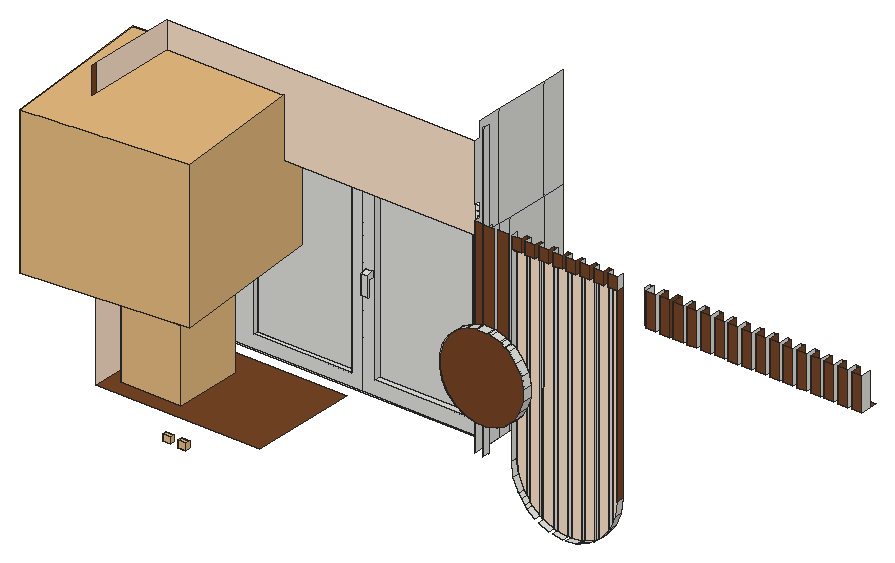
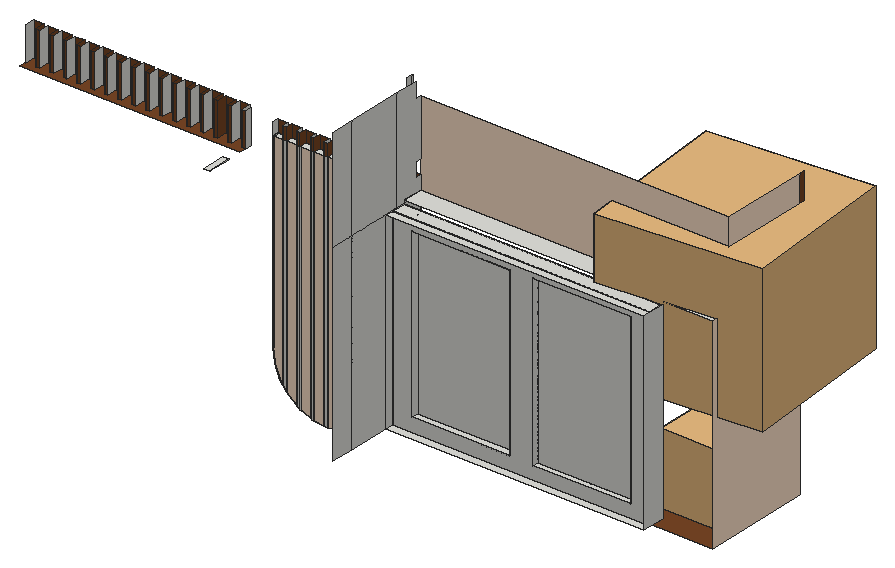
# SketchUp Ruby script. Lengths in inches.
U = 1.inch
M = Sketchup.active_model
def pt(a) = Geom::Point3d.new(a.map { |v| v * U })
def face(e, loops, mat)
  f = e.add_face(loops[0].map { |a| pt(a) })
  loops[1..].each { |l| e.add_face(l.map { |a| pt(a) }).erase! }
  f.material = f.back_material = mat if mat
  f
end
# faces: each face lists its corners as indices into pts; further lists are holes
def faces(e, pts, list, mat = nil) = list.each { |f| face(e, (f[0].is_a?(Array) ? f : [f]).map { |l| l.map { |i| pts[i] } }, mat) }
# xy, xz, yz: faces in a plane at the given z, y or x. An outline is a flat list of corners, or four numbers for a rectangle; further outlines are holes
def ring(l) = l.size == 4 ? [[l[0], l[1]], [l[2], l[1]], [l[2], l[3]], [l[0], l[3]]] : l.each_slice(2).to_a
def flat(e, list, mat, &to3) = list.each { |f| face(e, (f[0].is_a?(Array) ? f : [f]).map { |l| ring(l).map { |u, v| to3.(u, v) } }, mat) }
def xy(e, z, list, mat = nil) = flat(e, list, mat) { |x, y| [x, y, z] }
def xz(e, y, list, mat = nil) = flat(e, list, mat) { |x, z| [x, y, z] }
def yz(e, x, list, mat = nil) = flat(e, list, mat) { |y, z| [x, y, z] }
def lines(e, pts, list) = list.each { |a, b| e.add_line(pt(pts[a]), pt(pts[b])) }
# prism: a flat outline (further loops are holes) pulled along v
def prism(e, loops, v, mat = nil)
  f = face(e, loops, mat); d = Geom::Vector3d.new(v.map { |x| x * U })
  f.pushpull(f.normal.samedirection?(d) ? d.length : -d.length)
end
def box(e, o, s, mat = nil) = prism(e, [[o, [o[0] + s[0], o[1], o[2]], [o[0] + s[0], o[1] + s[1], o[2]], [o[0], o[1] + s[1], o[2]]]], [0, 0, s[2]], mat)
def at(x, y, z, deg = 0) = Geom::Transformation.translation(pt([x, y, z])) * Geom::Transformation.rotation(ORIGIN, Z_AXIS, deg.degrees)
def axes(o, x, y, z) = Geom::Transformation.new([*x, 0, *y, 0, *z, 0, *pt(o).to_a, 1])
def part(name) = M.definitions.add(name)
# library, detail: a bought-in or finely detailed component or shape, given as its bounding box
def library(name, o, s) = part(name).tap { |d| box(d.entities, o, s) }
def detail(e, o, s) = box(e.add_group.entities, o, s)
def put(e, d, t, mat = nil) = e.add_instance(d, t).tap { |i| i.material = mat if mat }
def group(e, t, mat = nil) = e.add_group.tap { |g| g.transformation = t; g.material = mat if mat }.entities
root = M.entities
M.materials.add("[Color C01]").color = [255, 229, 204]
M.materials.add("[Color M02]").color = [198, 198, 198]
M.materials.add("[Color M08]1").color = [30, 30, 30]
M.materials.add("[Wood Veneer 01]").color = [120, 70, 37]
c1 = library("Recessed spotlight",[0,0,0],[1.29,1.0625,0.73])
c2 = part("Window (3)")
xy(c2.entities,31.72,[[-0.78,88.6,2.72,128.1]])
xy(c2.entities,34.95,[[-0.78,91.53,0.84,106.59],[0.84,91.53,1.05,97.58],[1.05,91.53,1.42,106.59],[1.42,91.53,2.72,106.59],[0.84,97.58,1.05,98.18],
  [0.84,98.18,1.05,106.59]])
xy(c2.entities,35.27,[[-0.78,110.09,0.97,125.14],[1.05,110.09,2.72,125.14]])
xy(c2.entities,58.35,[[2.72,108.74,3.8,109.74]])
xy(c2.entities,77.8125,[[-0.78,110.09,2.72,125.14],[0.97,110.09,1.05,125.14]])
xy(c2.entities,77.93,[[-0.78,91.53,0.84,106.59],[1.05,91.53,1.42,106.59],[1.42,91.53,2.72,106.59]])
xy(c2.entities,80.72,[[-0.78,88.6,2.72,128.1]])
xz(c2.entities,88.6,[[-0.78,31.72,2.72,80.72]])
xz(c2.entities,91.53,[[-0.78,34.95,0.84,77.93],[1.05,34.95,1.42,77.93],[1.42,34.95,2.72,77.93]])
xz(c2.entities,106.59,[[-0.78,34.95,0.84,77.93],[0.84,34.95,1.05,77.93],[0.84,34.95,2.72,77.93]])
xz(c2.entities,108.74,[[3.8,54.35,4.22,54.6,4.22,59.47,2.72,59.97,2.72,58.35,3.8,58.35]])
xz(c2.entities,109.74,[[3.8,54.35,3.8,58.35,2.72,58.35,2.72,59.97,4.22,59.47,4.22,54.6]])
xz(c2.entities,110.09,[[-0.78,35.27,0.97,77.8125],[1.05,35.27,2.72,77.8125]])
xz(c2.entities,125.14,[[-0.78,35.27,0.97,77.8125],[0.97,35.27,1.05,80.72],[1.05,35.27,2.72,77.8125]])
xz(c2.entities,128.1,[[-0.78,31.72,2.72,80.72]])
yz(c2.entities,-0.78,[[[88.6,31.72,128.1,80.72],[91.53,34.95,106.59,77.93],[110.09,35.27,125.14,77.8125]]])
yz(c2.entities,0.84,[[91.53,34.95,106.59,77.93]])
yz(c2.entities,0.97,[[110.09,35.27,125.14,77.8125]])
yz(c2.entities,1.05,[[91.53,34.95,106.59,77.93],[110.09,35.27,125.14,77.8125]])
yz(c2.entities,1.42,[[91.53,34.95,106.59,77.93]])
yz(c2.entities,2.72,[[[88.6,31.72,108.35,80.72],[91.53,34.95,106.59,77.93]],[[108.35,31.72,128.1,80.72],[110.09,35.27,125.14,77.8125],[108.74,58.35,109.74,59.97]]])
yz(c2.entities,3.8,[[108.74,54.35,109.74,58.35]])
yz(c2.entities,4.22,[[108.74,54.6,109.74,59.47]])
p = [[4.22,108.74,54.6],[3.8,108.74,54.35],[3.8,109.74,54.35],[4.22,109.74,54.6],[2.72,109.74,59.97],[2.72,108.74,59.97],
  [4.22,108.74,59.47],[4.22,109.74,59.47],[-0.78,86.4,89.94],[-0.78,86.44,89.94],[15.22,130.69,89.94],[15.22,130.65,89.94],
  [-0.78,86.44,28.19],[-0.78,86.4,28.19],[7.72,130.69,89.94],[7.72,130.65,89.94]]
faces(c2.entities,p,[[0,1,2,3],[4,5,6,7]])
lines(c2.entities,p,[[8,9],[10,11],[12,13],[14,15]])
c3 = library("Potted plant pair",[-0.125,-0.11,0],[4.84,5.4,5.74])
c4 = library("Potted trailing plant",[-13.52,-13.75,-7.41],[40.56,40.5625,37.31])
xy(root,46.25,[[6.1,124.71,47.85,152.4]],"[Wood Veneer 01]")
xy(root,48.58,[[18.99,152.4,84.82,158.375]])
xy(root,50.17,[[94.24,147.02,94.43,148.71],[121.11,147.02,121.3,148.65],[121.11,148.65,121.3,148.71]])
xy(root,57.34,[[87.07,144.77,87.24,147.02]])
xy(root,91.72,[[129.68,152.25,131.15,158.375]])
xy(root,93.09,[[129.24,146.15,129.24,148.71,128.3,148.71,128.3,150.65,184.3,150.65,184.3,146.15,181.74,146.15,181.74,148.71,180.8,148.71,180.8,146.15,178.24,146.15,178.24,148.71,177.3,148.71,177.3,146.15,174.74,146.15,174.74,148.71,173.8,148.71,173.8,146.15,171.24,146.15,171.24,148.71,170.3,148.71,170.3,146.15,167.74,146.15,167.74,148.71,166.8,148.71,166.8,146.15,164.24,146.15,164.24,148.71,163.3,148.71,163.3,146.15,160.74,146.15,160.74,148.71,159.8,148.71,159.8,146.15,157.24,146.15,157.24,148.71,156.3,148.71,156.3,146.15,153.74,146.15,153.74,148.71,152.8,148.71,152.8,146.15,150.24,146.15,150.24,148.71,149.3,148.71,149.3,146.15,146.74,146.15,146.74,148.71,145.8,148.71,145.8,146.15,143.24,146.15,143.24,148.71,142.3,148.71,142.3,146.15,139.74,146.15,139.74,148.71,138.8,148.71,138.8,146.15,136.24,146.15,136.24,148.71,135.3,148.71,135.3,146.15,132.74,146.15,132.74,148.71,131.8,148.71,131.8,146.15]],"[Wood Veneer 01]")
xy(root,97.46,[[18.99,152.4,84.82,158.375]])
xy(root,98.3,[[6.1,147.26,84.82,152.4]])
xy(root,98.3,[[6.1,123.26,18.91,147.26]],"[Wood Veneer 01]")
xy(root,98.47,[[94.24,147.02,94.43,148.71],[94.43,147.02,96.8,148.65],[97.74,147.02,100.3,148.65],[101.24,147.02,103.8,148.65],[104.74,147.02,107.3,148.65],
  [108.24,147.02,110.8,148.65],[111.74,147.02,114.3,148.65],[115.24,147.02,117.8,148.65],[118.74,147.02,121.11,148.65],[121.11,147.02,121.3,148.71]])
xy(root,100.37,[[6.1,123.26,18.91,124.71],[6.1,124.71,18.91,147.26]])
xz(root,123.26,[[6.1,98.3,18.91,100.37]],"[Wood Veneer 01]")
xz(root,144.77,[[89.5,57.25,89.8,57.32,90.74,57.54,92.25,57.88,93.3,58.44,94.24,58.94,94.43,59.04,94.74,59.2,96.8,61.125,98.3,63.51,99.13,66.21,99.23,69.03,98.6,71.77,97.28,74.26,95.36,76.33,94.43,76.91,94.24,77.03,93.3,77.62,92.97,77.83,90.74,78.51,90.28,78.66,89.8,78.67,87.46,78.76,87.24,78.71,87.07,78.67,84.82,78.15,84.71,78.13,82.22,76.81,80.16,74.89,78.66,72.5,77.83,69.81,77.73,66.99,78.36,64.24,79.68,61.75,81.6,59.68,83.98,58.1875,84.82,57.93,86.68,57.36,87.07,57.34,87.24,57.34]],"[Wood Veneer 01]")
xz(root,146.15,[[129.24,93.09,131.8,101.64],[132.74,93.09,135.3,101.64],[136.24,93.09,138.8,101.64],[139.74,93.09,142.3,101.64],[143.24,93.09,145.8,101.64],
  [146.74,93.09,149.3,101.64],[150.24,93.09,152.8,101.64],[153.74,93.09,156.3,101.64],[157.24,93.09,159.8,101.64],[160.74,93.09,163.3,101.64],
  [164.24,93.09,166.8,101.64],[167.74,93.09,170.3,101.64],[171.24,93.09,173.8,101.64],[174.74,93.09,177.3,101.64],[178.24,93.09,180.8,101.64],
  [181.74,93.09,184.3,101.64]],"[Wood Veneer 01]")
xz(root,147.02,[[110.8,37.04,111.74,37.3,114.3,38.36],[94.24,50.17,94.43,50.17,94.43,59.04,94.24,58.94],[121.11,50.17,121.3,98.47],[89.8,57.32,89.8,78.67,90.28,78.66,90.74,78.51,90.74,57.54],[87.07,57.34,87.07,78.67,87.24,78.71,87.24,57.34],
  [84.82,57.93,83.98,58.1875,81.6,59.68,79.68,61.75,78.36,64.24,77.73,66.99,77.83,69.81,78.66,72.5,80.16,74.89,82.22,76.81,84.71,78.13,84.82,78.15],[93.3,58.44,93.3,77.62,94.24,77.03,94.24,58.94],[94.43,59.04,94.43,76.91,95.36,76.33,97.28,74.26,98.6,71.77,99.23,69.03,99.13,66.21,98.3,63.51,96.8,61.125,94.74,59.2],[94.43,76.91,94.43,98.47,94.24,98.47,94.24,77.03]])
xz(root,147.02,[[93.3,77.62,93.3,101.64,90.74,101.64,90.74,78.51,92.97,77.83],[84.82,78.15,87.07,78.67,87.07,101.64,84.82,101.64],[89.8,78.67,89.8,101.64,87.24,101.64,87.24,78.71,87.46,78.76],[94.24,98.47,96.8,101.64],[97.74,98.47,100.3,101.64],
  [101.24,98.47,103.8,101.64],[104.74,98.47,107.3,101.64],[108.24,98.47,110.8,101.64],[111.74,98.47,114.3,101.64],[115.24,98.47,117.8,101.64],
  [118.74,98.47,121.3,101.64]],"[Wood Veneer 01]")
xz(root,147.26,[[18.91,98.3,84.82,98.3,84.82,119.8125,6.1,119.8125,6.1,100.37,18.91,100.37]],"[Color C01]")
xz(root,148.65,[[107.3,36.71,107.3,98.47,104.74,98.47,104.74,37.04],[108.24,36.71,110.8,37.04,110.8,98.47,108.24,98.47],[103.8,37.3,103.8,98.47,101.24,98.47,101.01,38.46,101.24,38.36],[111.74,37.3,114.3,38.36,114.3,98.47,111.74,98.47],[100.3,39,100.3,98.47,97.74,98.47,97.74,41.21,98.21,40.61],
  [115.24,39,117.34,40.61,117.8,41.21,117.8,98.47,115.24,98.47],[96.8,42.4375,96.8,98.47,94.43,98.47,94.43,48.75,94.71,46.67,96.06,43.41],[118.74,42.4375,119.49,43.41,120.84,46.67,121.3,50.17,121.11,50.17,121.11,98.47,118.74,98.47]],"[Color C01]")
xz(root,148.71,[[107.77,36.64,108.24,36.71,108.24,98.47,107.3,98.47,107.3,36.71],[104.74,37.04,104.74,98.47,103.8,98.47,103.8,37.3,104.27,37.1],[110.8,37.04,111.27,37.1,111.74,37.3,111.74,98.47,110.8,98.47],[114.3,38.36,114.54,38.46,115.24,39,115.24,98.47,114.3,98.47],[101.01,38.46,101.24,98.47,100.3,98.47,100.3,39],
  [97.74,41.21,97.74,98.47,96.8,98.47,96.8,42.4375],[117.8,41.21,118.74,42.4375,118.74,98.47,117.8,98.47],[94.43,42.4375,96.8,42.4375,96.06,43.41,94.71,46.67,94.43,48.75],[87.07,48.58,87.24,97.46],[94.43,48.75,94.43,50.17,94.24,50.17],
  [94.24,50.17,94.43,98.47],[121.11,50.17,121.3,98.47],[87.07,97.46,87.24,101.64]])
xz(root,148.71,[[128.3,93.09,129.24,101.64],[131.8,93.09,132.74,101.64],[135.3,93.09,136.24,101.64],[138.8,93.09,139.74,101.64],[142.3,93.09,143.24,101.64],
  [145.8,93.09,146.74,101.64],[149.3,93.09,150.24,101.64],[152.8,93.09,153.74,101.64],[156.3,93.09,157.24,101.64],[159.8,93.09,160.74,101.64],
  [163.3,93.09,164.24,101.64],[166.8,93.09,167.74,101.64],[170.3,93.09,171.24,101.64],[173.8,93.09,174.74,101.64],[177.3,93.09,178.24,101.64],
  [180.8,93.09,181.74,101.64],[96.8,98.47,97.74,101.64],[100.3,98.47,101.24,101.64],[103.8,98.47,104.74,101.64],[107.3,98.47,108.24,101.64],
  [110.8,98.47,111.74,101.64],[114.3,98.47,115.24,101.64],[117.8,98.47,118.74,101.64]],"[Wood Veneer 01]")
yz(root,6.1,[[124.71,46.25,152.4,98.3],[124.71,100.37,147.26,119.8125]],"[Color C01]")
yz(root,6.1,[[123.26,100.37,124.71,119.8125]],"[Wood Veneer 01]")
yz(root,18.91,[[123.26,98.3,147.26,100.37]],"[Wood Veneer 01]")
yz(root,18.99,[[152.4,48.58,158.375,97.46]])
yz(root,84.82,[[147.02,48.58,147.26,97.46],[147.26,48.58,154.8125,97.46],[154.8125,48.58,158.375,97.46],[158.375,48.58,169.1875,97.46],[169.1875,48.58,175.3125,97.46],
  [147.02,97.46,147.26,101.64],[147.26,97.46,152.4,98.3],[152.4,97.46,152.4,98.3,147.26,98.3,147.26,101.64,148.71,101.64,148.71,105.33,147.26,105.33,147.26,119.8125,148.71,119.8125,148.71,123.71,154.8125,123.71,154.8125,97.46],[154.8125,97.46,169.1875,123.71],[169.1875,97.46,175.3125,123.71]])
yz(root,87.07,[[147.02,48.58,147.26,97.46],[147.26,48.58,148.71,97.46],[147.02,97.46,147.26,123.71],[147.26,97.46,148.71,123.71]])
yz(root,94.24,[[147.02,98.47,148.71,101.64]])
yz(root,94.24,[[147.02,50.17,148.71,98.47]],"[Wood Veneer 01]")
yz(root,94.43,[[148.65,48.75,148.71,50.17],[147.02,50.17,148.65,98.47],[148.65,50.17,148.71,98.47]])
yz(root,96.8,[[148.65,42.4375,148.71,98.47]])
yz(root,96.8,[[147.02,98.47,148.71,101.64]],"[Wood Veneer 01]")
yz(root,97.74,[[148.65,41.21,148.71,98.47],[147.02,98.47,148.71,101.64]])
yz(root,100.3,[[148.65,39,148.71,98.47]])
yz(root,100.3,[[147.02,98.47,148.71,101.64]],"[Wood Veneer 01]")
yz(root,101.24,[[147.02,98.47,148.71,101.64]])
yz(root,103.8,[[148.65,37.3,148.71,98.47]])
yz(root,103.8,[[147.02,98.47,148.71,101.64]],"[Wood Veneer 01]")
yz(root,104.74,[[148.65,37.04,148.71,98.47],[147.02,98.47,148.71,101.64]])
yz(root,107.3,[[148.65,36.71,148.71,37.04],[148.65,37.04,148.71,98.47]])
yz(root,107.3,[[147.02,98.47,148.71,101.64]],"[Wood Veneer 01]")
yz(root,108.24,[[148.65,36.71,148.71,98.47],[147.02,98.47,148.71,101.64]])
yz(root,110.8,[[148.65,37.04,148.71,98.47]])
yz(root,110.8,[[147.02,98.47,148.71,101.64]],"[Wood Veneer 01]")
yz(root,111.74,[[148.65,37.3,148.71,98.47],[147.02,98.47,148.71,101.64]])
yz(root,114.3,[[148.65,38.36,148.71,98.47]])
yz(root,114.3,[[147.02,98.47,148.71,101.64]],"[Wood Veneer 01]")
yz(root,115.24,[[148.65,39,148.71,98.47],[147.02,98.47,148.71,101.64]])
yz(root,117.8,[[148.65,41.21,148.71,98.47]])
yz(root,117.8,[[147.02,98.47,148.71,101.64]],"[Wood Veneer 01]")
yz(root,118.74,[[148.65,42.4375,148.71,98.47],[147.02,98.47,148.71,101.64]])
yz(root,121.11,[[147.02,50.17,148.65,98.47],[148.65,50.17,148.71,98.47]])
yz(root,121.3,[[147.02,98.47,148.71,101.64]])
yz(root,121.3,[[147.02,50.17,148.71,98.47]],"[Wood Veneer 01]")
yz(root,128.3,[[147.02,93.09,148.71,101.64]])
yz(root,129.24,[[146.15,93.09,148.71,101.64]])
yz(root,129.68,[[152.25,91.66,158.375,91.72]])
yz(root,131.8,[[146.15,93.09,148.71,101.64]])
yz(root,132.74,[[146.15,93.09,148.71,101.64]],"[Wood Veneer 01]")
yz(root,135.3,[[146.15,93.09,148.71,101.64]],"[Wood Veneer 01]")
yz(root,136.24,[[146.15,93.09,148.71,101.64]],"[Wood Veneer 01]")
yz(root,138.8,[[146.15,93.09,148.71,101.64]])
yz(root,139.74,[[146.15,93.09,148.71,101.64]],"[Wood Veneer 01]")
yz(root,142.3,[[146.15,93.09,148.71,101.64]])
yz(root,143.24,[[146.15,93.09,148.71,101.64]],"[Wood Veneer 01]")
yz(root,145.8,[[146.15,93.09,148.71,101.64]])
yz(root,146.74,[[146.15,93.09,148.71,101.64]],"[Wood Veneer 01]")
yz(root,149.3,[[146.15,93.09,148.71,101.64]])
yz(root,150.24,[[146.15,93.09,148.71,101.64]],"[Wood Veneer 01]")
yz(root,152.8,[[146.15,93.09,148.71,101.64]])
yz(root,153.74,[[146.15,93.09,148.71,101.64]],"[Wood Veneer 01]")
yz(root,156.3,[[146.15,93.09,148.71,101.64]])
yz(root,157.24,[[146.15,93.09,148.71,101.64]],"[Wood Veneer 01]")
yz(root,159.8,[[146.15,93.09,148.71,101.64]])
yz(root,160.74,[[146.15,93.09,148.71,101.64]],"[Wood Veneer 01]")
yz(root,163.3,[[146.15,93.09,148.71,101.64]])
yz(root,164.24,[[146.15,93.09,148.71,101.64]],"[Wood Veneer 01]")
yz(root,166.8,[[146.15,93.09,148.71,101.64]])
yz(root,167.74,[[146.15,93.09,148.71,101.64]],"[Wood Veneer 01]")
yz(root,170.3,[[146.15,93.09,148.71,101.64]])
yz(root,171.24,[[146.15,93.09,148.71,101.64]],"[Wood Veneer 01]")
yz(root,173.8,[[146.15,93.09,148.71,101.64]])
yz(root,174.74,[[146.15,93.09,148.71,101.64]],"[Wood Veneer 01]")
yz(root,177.3,[[146.15,93.09,148.71,101.64]])
yz(root,178.24,[[146.15,93.09,148.71,101.64]],"[Wood Veneer 01]")
yz(root,180.8,[[146.15,93.09,148.71,101.64]])
yz(root,181.74,[[146.15,93.09,148.71,101.64]],"[Wood Veneer 01]")
yz(root,184.3,[[146.15,93.09,148.71,101.64]])
p = [[107.3,147.02,36.71],[107.3,148.65,36.71],[104.74,148.65,37.04],[104.74,147.02,37.04],[110.8,147.02,37.04],[110.8,148.65,37.04],
  [108.24,148.65,36.71],[108.24,147.02,36.71],[103.8,147.02,37.3],[103.8,148.65,37.3],[101.24,148.65,38.36],[101.24,147.02,38.36],
  [114.3,147.02,38.36],[114.3,148.65,38.36],[111.74,148.65,37.3],[111.74,147.02,37.3],[101.01,148.71,38.46],[101.24,148.71,38.36],
  [101.01,148.65,38.46],[101.24,148.71,98.47],[101.24,148.65,98.47],[100.3,147.02,39],[100.3,148.65,39],[98.21,148.65,40.61],
  [98.21,147.02,40.61],[117.34,147.02,40.61],[117.34,148.65,40.61],[115.24,148.65,39],[115.24,147.02,39],[97.74,148.65,41.21],
  [97.74,147.02,41.21],[117.8,147.02,41.21],[117.8,148.65,41.21],[96.8,147.02,42.4375],[97.74,148.71,41.21],[96.8,148.71,42.4375],
  [96.8,148.65,42.4375],[118.74,147.02,42.4375],[118.74,148.65,42.4375],[118.74,148.71,42.4375],[117.8,148.71,41.21],[96.06,148.65,43.41],
  [96.06,147.02,43.41],[119.49,147.02,43.41],[119.49,148.65,43.41],[96.06,148.71,43.41],[94.71,148.65,46.67],[94.71,147.02,46.67],
  [120.84,147.02,46.67],[120.84,148.65,46.67],[94.71,148.71,46.67],[94.43,148.71,48.75],[94.24,148.71,50.17],[94.24,147.02,50.17],
  [94.43,148.65,48.75],[121.3,147.02,50.17],[121.3,148.65,50.17],[86.68,147.02,57.36],[87.07,147.02,57.34],[87.07,144.77,57.34],
  [86.68,144.77,57.36],[87.24,147.02,57.34],[89.5,147.02,57.25],[89.5,144.77,57.25],[87.24,144.77,57.34],[89.8,147.02,57.32],
  [89.8,144.77,57.32],[90.74,147.02,57.54],[90.74,144.77,57.54],[84.82,147.02,57.93],[84.82,144.77,57.93],[92.25,147.02,57.88],
  [92.25,144.77,57.88],[83.98,147.02,58.1875],[83.98,144.77,58.1875],[93.3,147.02,58.44],[93.3,144.77,58.44],[81.6,147.02,59.68],
  [81.6,144.77,59.68],[94.24,147.02,58.94],[94.24,144.77,58.94],[94.43,147.02,59.04],[94.43,144.77,59.04],[94.74,147.02,59.2],
  [94.74,144.77,59.2],[96.8,147.02,61.125],[96.8,144.77,61.125],[79.68,147.02,61.75],[79.68,144.77,61.75],[98.3,147.02,63.51],
  [98.3,144.77,63.51],[78.36,147.02,64.24],[78.36,144.77,64.24],[99.13,147.02,66.21],[99.13,144.77,66.21],[77.73,147.02,66.99],
  [77.73,144.77,66.99],[99.23,147.02,69.03],[99.23,144.77,69.03],[77.83,147.02,69.81],[77.83,144.77,69.81],[98.6,147.02,71.77],
  [98.6,144.77,71.77],[78.66,147.02,72.5],[78.66,144.77,72.5],[97.28,147.02,74.26],[97.28,144.77,74.26],[80.16,147.02,74.89],
  [80.16,144.77,74.89],[95.36,147.02,76.33],[95.36,144.77,76.33],[82.22,147.02,76.81],[82.22,144.77,76.81],[94.43,147.02,76.91],
  [94.43,144.77,76.91],[84.71,147.02,78.13],[84.71,144.77,78.13],[94.24,147.02,77.03],[94.24,144.77,77.03],[93.3,147.02,77.62],
  [93.3,144.77,77.62],[92.97,147.02,77.83],[92.97,144.77,77.83],[90.74,147.02,78.51],[90.74,144.77,78.51],[84.82,147.02,78.15],
  [84.82,144.77,78.15],[87.07,147.02,78.67],[87.07,144.77,78.67],[90.28,147.02,78.66],[90.28,144.77,78.66],[87.24,147.02,78.71],
  [87.24,144.77,78.71],[87.46,147.02,78.76],[87.46,144.77,78.76],[89.8,147.02,78.67],[89.8,144.77,78.67]]
faces(root,p,[[0,1,2,3],[4,5,6,7],[8,9,10,11],[12,13,14,15],[16,17,10,18],[19,16,18,20],[21,22,23,24],[25,26,27,28],
  [24,23,29,30],[31,32,26,25],[33,30,29,34,35,36],[31,37,38,39,40,32],[33,36,41,42],[43,44,38,37],[35,45,41,36],[42,41,46,47],
  [48,49,44,43],[45,50,46,41],[51,52,53,47,46,54],[55,56,49,48],[50,51,54,46],[57,58,59,60],[61,62,63,64],[62,65,66,63],
  [65,67,68,66],[69,57,60,70],[67,71,72,68],[73,69,70,74],[71,75,76,72],[77,73,74,78],[75,79,80,76],[79,81,82,80],
  [81,83,84,82],[83,85,86,84],[87,77,78,88],[85,89,90,86],[91,87,88,92],[89,93,94,90],[95,91,92,96],[93,97,98,94],
  [99,95,96,100],[97,101,102,98],[103,99,100,104],[101,105,106,102],[107,103,104,108],[105,109,110,106],[111,107,108,112],[109,113,114,110],
  [115,111,112,116],[113,117,118,114],[117,119,120,118],[119,121,122,120],[121,123,124,122],[125,115,116,126],[127,125,126,128],[123,129,130,124],
  [131,127,128,132],[133,131,132,134],[135,133,134,136],[129,135,136,130]])
lines(root,p,[[21,11],[3,8],[0,7],[28,12]])
put(root,c1,axes([23.99,124.71,40.21],[1.55,0,0],[0,0,1.55],[0,-1.55,0]),"[Color M08]1")
put(root,c1,axes([27.99,124.71,40.21],[1.55,0,0],[0,0,1.55],[0,-1.55,0]),"[Color M08]1")
put(root,c2,axes([-128.01,155.55,16.86],[0,-1,0],[1.65965,0,0],[0,0,1]))
put(root,c3,axes([9.54,129.11,46.25],[3.18,0,0],[0,3.18,0],[0,0,3.18]),"[Color C01]")
put(root,c4,at(24.08,125.7,83.22,95.1),"[Color M02]")
